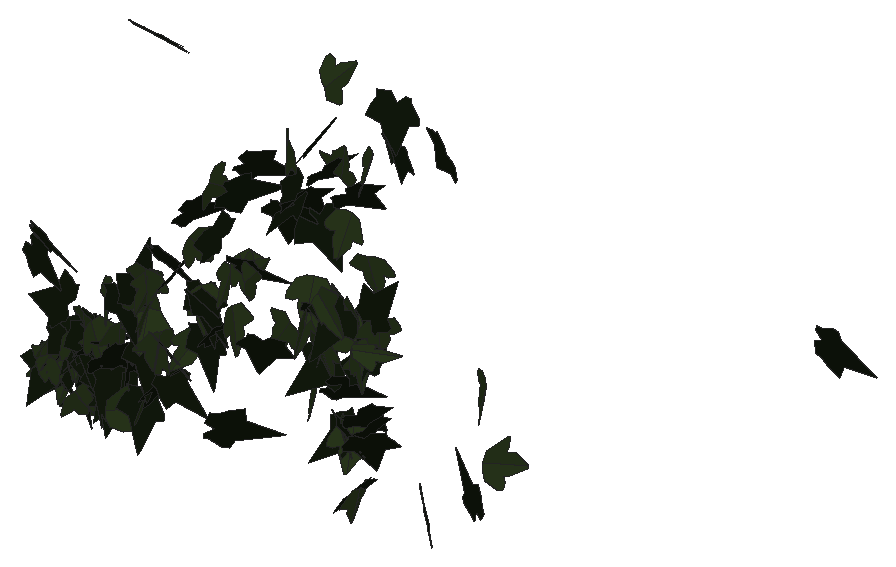
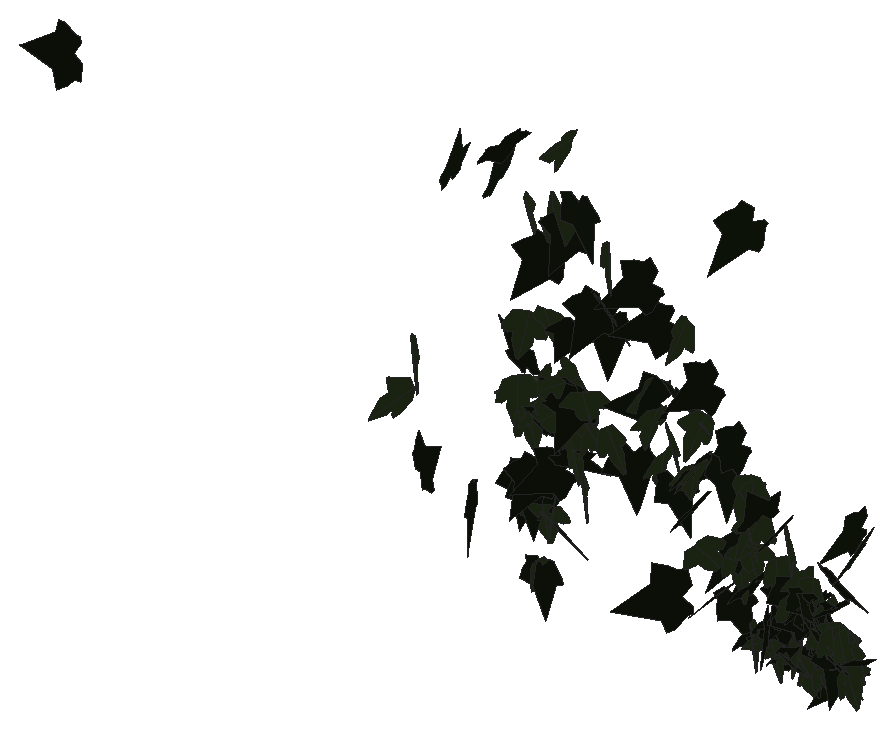
# SketchUp Ruby script. Lengths in inches.
U = 1.inch
M = Sketchup.active_model
def pt(a) = Geom::Point3d.new(a.map { |v| v * U })
def face(e, loops, mat)
  f = e.add_face(loops[0].map { |a| pt(a) })
  loops[1..].each { |l| e.add_face(l.map { |a| pt(a) }).erase! }
  f.material = f.back_material = mat if mat
  f
end
# faces: each face lists its corners as indices into pts; further lists are holes
def faces(e, pts, list, mat = nil) = list.each { |f| face(e, (f[0].is_a?(Array) ? f : [f]).map { |l| l.map { |i| pts[i] } }, mat) }
# xy, xz, yz: faces in a plane at the given z, y or x. An outline is a flat list of corners, or four numbers for a rectangle; further outlines are holes
def ring(l) = l.size == 4 ? [[l[0], l[1]], [l[2], l[1]], [l[2], l[3]], [l[0], l[3]]] : l.each_slice(2).to_a
def flat(e, list, mat, &to3) = list.each { |f| face(e, (f[0].is_a?(Array) ? f : [f]).map { |l| ring(l).map { |u, v| to3.(u, v) } }, mat) }
def xy(e, z, list, mat = nil) = flat(e, list, mat) { |x, y| [x, y, z] }
def xz(e, y, list, mat = nil) = flat(e, list, mat) { |x, z| [x, y, z] }
def yz(e, x, list, mat = nil) = flat(e, list, mat) { |y, z| [x, y, z] }
def lines(e, pts, list) = list.each { |a, b| e.add_line(pt(pts[a]), pt(pts[b])) }
# prism: a flat outline (further loops are holes) pulled along v
def prism(e, loops, v, mat = nil)
  f = face(e, loops, mat); d = Geom::Vector3d.new(v.map { |x| x * U })
  f.pushpull(f.normal.samedirection?(d) ? d.length : -d.length)
end
def box(e, o, s, mat = nil) = prism(e, [[o, [o[0] + s[0], o[1], o[2]], [o[0] + s[0], o[1] + s[1], o[2]], [o[0], o[1] + s[1], o[2]]]], [0, 0, s[2]], mat)
def at(x, y, z, deg = 0) = Geom::Transformation.translation(pt([x, y, z])) * Geom::Transformation.rotation(ORIGIN, Z_AXIS, deg.degrees)
def axes(o, x, y, z) = Geom::Transformation.new([*x, 0, *y, 0, *z, 0, *pt(o).to_a, 1])
def part(name) = M.definitions.add(name)
# library, detail: a bought-in or finely detailed component or shape, given as its bounding box
def library(name, o, s) = part(name).tap { |d| box(d.entities, o, s) }
def detail(e, o, s) = box(e.add_group.entities, o, s)
def put(e, d, t, mat = nil) = e.add_instance(d, t).tap { |i| i.material = mat if mat }
def group(e, t, mat = nil) = e.add_group.tap { |g| g.transformation = t; g.material = mat if mat }.entities
root = M.entities
M.materials.add("efeu1").color = [18, 25, 13]
M.materials.add("efeu2").color = [43, 57, 29]
c1 = part("ivyleaf_9")
p = [[1.54,2.16,1.25],[1.36,2.04,1.19],[-0.21,0.99,0.68],[-0.71,1.11,0.82],[-0.85,0.86,0.67],[-0.8,0.17,0.21],
  [-0.9,-0.01,0.1],[-0.67,-0.16,-0.02],[-0.08,-0.08,-0.05],[-0.03,-0.6,-0.4],[0.65,-0.88,-0.66],[0.83,-0.6,-0.49],
  [1.29,-0.42,-0.43],[1.8125,-0.07,-0.26],[1.21,0.44,0.15]]
faces(c1.entities,p,[[0,1,2,3,4,5,6,7,8,9,10,11,12,13,14]],"efeu1")
c2 = part("ivyleaf_10")
p = [[0,0.5,-0.03],[-0.0625,2.02,-0.43],[-0.19,2.01,-0.46],[-0.54,1.05,-0.29],[-0.52,0.625,-0.18],[-0.83,0.76,-0.28],
  [-1.16,0.64,-0.33],[-1.15,0.33,-0.24],[-0.77,-0.39,0.02],[-0.3,-0.51,0.16],[0.04,-0.48,0.23],[-0.02,2.01,-0.4375],
  [-0.06,2.01,-0.43],[0.04,-0.49,0.23],[0.67,-0.49,0.14],[1.38,0.36,-0.2],[1.375,0.51,-0.24],[0.81,0.65,-0.19],
  [0.62,0.59,-0.15],[0.6,1.09,-0.28],[0.5,1.23,-0.31]]
faces(c2.entities,p,[[0,1,2,3,4,5,6,7,8,9,10],[11,12,0,13,14,15,16,17,18,19,20]],"efeu2")
put(root,c1,axes([585.08,129.7,253.83],[1.04572,-0.05683,0.01946],[0.02203,0.04717,-1.04615],[0.05589,1.04484,0.04829]))
put(root,c2,axes([579.78,129.68,243.31],[-0.42415,-0.71462,-0.56248],[0.29905,0.47653,-0.83094],[0.85886,-0.51885,0.01155]))
put(root,c1,axes([587.74,130.46,249.34],[0.2356,-1.00803,0.0812],[0.02153,-0.07835,-1.03519],[1.01106,0.23656,0.00312]))
put(root,c2,axes([577.44,130.0625,244.39],[-0.84516,0.20624,0.52283],[-0.55979,-0.22451,-0.81634],[-0.05023,-0.96811,0.30069]))
put(root,c2,axes([595.76,130.15,254.29],[0.58897,0.00063,0.92492],[0.92487,0.01136,-0.58895],[-0.00992,1.09647,0.00557]))
put(root,c1,axes([592.11,129.78,250.8],[0.56686,0.68354,-0.59156],[-0.4325,-0.40807,-0.88596],[-0.7938,0.71046,0.06028]))
put(root,c1,axes([595.93,129.64,264.52],[-0.36405,1.05527,0.03181],[-0.00822,0.03081,-1.1163],[-1.05572,-0.36413,-0.00228]))
put(root,c2,axes([597.04,130.17,262.6],[-1.0381,0.08365,0.31829],[0.31731,-0.02495,1.04146],[0.08729,1.08551,-0.00059]))
put(root,c1,axes([578.63,130.28,246.41],[0.17103,-0.97793,-0.23774],[0.18827,0.26798,-0.96689],[0.98865,0.11815,0.22525]))
put(root,c2,axes([589.98,130.03,251.53],[-0.04841,1.04429,-0.13892],[0.00143,-0.13901,-1.0454],[-1.05349,-0.04818,0.00497]))
put(root,c2,axes([579.11,130.05,246.22],[0.0865,1.01039,-0.14055],[-0.02968,-0.13851,-1.01393],[-1.01968,0.08974,0.01759]))
put(root,c1,axes([584.63,129.36,267.26],[1.15865,0.34915,-0.23864],[-0.33283,0.32341,-1.14278],[-0.26092,1.13791,0.39802]))
put(root,c2,axes([580.74,129.8125,247.49],[0.01702,1.01449,0.18738],[-0.05066,0.188,-1.01325],[-1.0304,0.00751,0.05291]))
put(root,c2,axes([598.9,129.65,252.64],[0.66546,-0.78164,-0.07907],[0.78558,0.66311,0.05651],[0.00802,-0.09685,1.02499]))
put(root,c2,axes([583.99,130.6,251.39],[-0.01699,-0.87816,0.53969],[0.06668,-0.53957,-0.87586],[1.02858,0.02047,0.0657]))
put(root,c2,axes([588.93,129.52,259.43],[-0.03718,-0.63777,-0.85772],[0.11562,0.8508,-0.63764],[1.06257,-0.11489,0.03937]))
put(root,c1,axes([596.79,130.59,253.92],[-0.95992,-0.43922,-0.12493],[0.13077,0.01423,-1.05483],[0.43752,-0.96791,0.04118]))
put(root,c2,axes([584.14,130.0625,251.92],[-1.01434,-0.05409,0.16911],[-0.16615,-0.05661,-1.01469],[0.06259,-1.02678,0.04703]))
put(root,c1,axes([600.4,130.87,265.06],[0.17117,-0.7786,0.7468],[0.23075,-0.71222,-0.79544],[1.05389,0.2824,0.05287]))
put(root,c1,axes([576.52,129.99,250.92],[0.7137,-0.62816,-0.42994],[-0.25555,0.35743,-0.94643],[0.71702,0.75264,0.09063]))
put(root,c1,axes([581.13,130.66,244.72],[-0.24631,-0.97162,-0.0316],[0.00525,0.03127,-1.00235],[0.97212,-0.24635,-0.0026]))
put(root,c1,axes([596.55,129.41,262.91],[0.40146,0.95016,0.32318],[0.02996,0.33657,-1.02676],[-1.00317,0.39029,0.09867]))
put(root,c1,axes([582.04,130.47,249.91],[0.3517,-0.97481,-0.06017],[0.01617,0.06975,-1.03559],[0.97653,0.34992,0.03882]))
put(root,c1,axes([591.25,129.58,261.37],[0.80293,0.40631,0.56612],[0.51853,0.22863,-0.89952],[-0.46552,0.95547,-0.02549]))
put(root,c1,axes([599.04,129.8,247.32],[0.61441,0.79835,-0.297],[-0.17054,-0.2435,-1.00732],[-0.83456,0.63751,-0.01282]))
put(root,c2,axes([591.43,129.4,254.64],[0.10894,-0.01752,-1.05804],[0.07748,1.06091,-0.00959],[1.05534,-0.07608,0.10993]))
put(root,c1,axes([603.02,129.72,244.72],[0.473,-0.04615,-1.08266],[-1.05154,0.26586,-0.47074],[0.26181,1.15117,0.06531]))
put(root,c1,axes([587.52,130.37,251.75],[0.55737,-0.87545,-0.09952],[0.04791,0.14771,-1.03096],[0.87978,0.54658,0.1192]))
put(root,c1,axes([581.1,130.91,243.53],[-0.03524,-0.94211,0.37102],[0.07599,-0.37265,-0.93905],[1.00968,-0.00484,0.08362]))
put(root,c2,axes([583.86,130.29,249.78],[0.44977,-0.9049,-0.16697],[-0.09992,0.13672,-1.01012],[0.91474,0.45987,-0.02824]))
put(root,c1,axes([587.59,130.56,251.92],[0.19776,-1.00869,-0.13422],[-0.04239,0.12845,-1.02775],[1.01669,0.20156,-0.01675]))
put(root,c2,axes([598.74,130.37,263.73],[0.6375,-0.86934,-0.08392],[-0.05647,0.06265,-1.078],[0.87156,0.63994,-0.00847]))
put(root,c1,axes([590.33,130,254.66],[0.83608,-0.20903,0.61257],[0.63719,0.09002,-0.83896],[0.11371,1.03255,0.19715]))
put(root,c1,axes([590.18,129.49,259.35],[0.09954,0.53535,-0.92841],[0.13362,0.91894,0.54421],[1.06334,-0.16559,0.01853]))
put(root,c1,axes([588.97,130.07,255.82],[-0.64361,0.73023,0.38332],[-0.36076,0.18796,-0.96381],[-0.74164,-0.72514,0.13619]))
put(root,c1,axes([579.84,130.77,246.82],[-0.93479,-0.41363,-0.06479],[0.06117,0.02188,-1.0222],[0.41418,-0.93678,0.00474]))
put(root,c1,axes([579.65,130.76,246.53],[0.01366,-1.02388,-0.05878],[0.03218,0.05919,-1.02344],[1.02506,0.01178,0.03292]))
put(root,c1,axes([583.26,130.87,243.73],[-0.11947,-1.01271,0.05879],[-0.02267,-0.05652,-1.01961],[1.01416,-0.12056,-0.01587]))
put(root,c1,axes([576.6875,130.11,251.93],[0.96616,-0.36901,-0.14248],[-0.08239,0.18005,-1.02505],[0.38688,0.95987,0.1375]))
put(root,c1,axes([577.08,131.05,243.83],[-0.60378,-0.78567,0.20996],[0.02508,-0.27937,-0.97327],[0.81286,-0.57497,0.18599]))
put(root,c1,axes([578.55,130.1,248.2],[-0.61269,0.52484,0.67507],[-0.54767,0.39692,-0.80565],[-0.65668,-0.82071,0.04206]))
put(root,c1,axes([581.46,129.69,246.24],[0.39769,0.89977,0.25094],[0.12839,0.21749,-0.98333],[-0.92525,0.41692,-0.02859]))
put(root,c2,axes([581.14,130.5,249.875],[0.73225,-0.7306,0.07881],[0.15734,0.0472,-1.0243],[0.7178,0.73496,0.14412]))
put(root,c2,axes([587.62,130.35,251.8],[0.24925,1.00951,-0.07355],[-0.00894,-0.07355,-1.03979],[-1.01215,0.24925,-0.00893]))
put(root,c1,axes([589.03,130.15,250.5],[-0.22262,0.99718,-0.24179],[0.00178,-0.24704,-1.02046],[-1.02607,-0.21677,0.05069]))
put(root,c1,axes([596.99,131,246.5],[0.83591,-0.58108,-0.25404],[0.20113,-0.15571,1.01796],[-0.60145,-0.85968,-0.01266]))
put(root,c2,axes([581.96,130.4,247.83],[-0.11576,-0.99997,-0.13419],[0.02572,0.13211,-1.0066],[1.00861,-0.11813,0.01026]))
put(root,c2,axes([582.32,129.7,243.26],[-0.00009,0.02567,1.05537],[0.27659,1.0185,-0.02475],[-1.0188,0.27651,-0.00681]))
put(root,c1,axes([580.97,130.03,246.79],[0.19064,0.97908,-0.1769],[-0.13942,-0.15205,-0.9918],[-0.98511,0.21099,0.10614]))
put(root,c2,axes([589.08,130.53,253.38],[0.75306,-0.70421,-0.13856],[-0.08763,0.10911,-1.03084],[0.71234,0.75788,0.01966]))
put(root,c2,axes([598.07,130.45,252],[-0.09724,1.07,-0.13702],[-0.00038,-0.13761,-1.07433],[-1.07874,-0.09641,0.01273]))
put(root,c2,axes([593.25,130.47,251.82],[-0.80962,0.11397,0.63442],[-0.64457,-0.1419,-0.79708],[-0.00079,-1.01874,0.182]))
put(root,c2,axes([607.75,129.65,248.98],[-0.0138,0.37019,1.08543],[0.0478,1.08475,-0.36935],[-1.14583,0.04079,-0.02848]))
put(root,c2,axes([595.6,130.35,251.69],[-1.01493,0.36891,-0.06535],[0.07019,0.00184,-1.07959],[-0.36802,-1.01703,-0.02566]))
put(root,c1,axes([584.77,130.24,248.01],[0.98072,-0.12195,-0.2982],[-0.28528,0.11525,-0.98536],[0.1497,1.01855,0.07579]))
put(root,c1,axes([600.05,131.09,267.34],[-0.12461,-1.08112,-0.01233],[-0.01195,0.01379,-1.08819],[1.08112,-0.12446,-0.01345]))
put(root,c1,axes([586.94,129.75,256.83],[0.5554,0.58339,0.68873],[0.43171,0.53848,-0.80426],[-0.79266,0.70204,0.04456]))
put(root,c1,axes([598.84,130.54,254.29],[-0.43848,0.42566,0.83574],[0.59286,-0.58907,0.61108],[0.72674,0.73737,0.00573]))
put(root,c2,axes([595.02,130.41,248.59],[0.5666,-0.80732,-0.46619],[-0.1904,0.43383,-0.98269],[0.91261,0.59175,0.08442]))
put(root,c1,axes([593.67,130.8,260.04],[-1.01077,0.26582,-0.2538],[0.25317,-0.0348,-1.04471],[-0.26642,-1.04156,-0.02987]))
put(root,c2,axes([584.34,130.72,247.89],[-0.34429,-0.9639,0.0793],[0.0129,-0.08874,-1.02269],[0.96707,-0.34198,0.04187]))
put(root,c1,axes([583.28,131.15,246.66],[-0.0083,-1.00964,0.10048],[0.05512,-0.10078,-1.00814],[1.01313,-0.00279,0.05567]))
put(root,c1,axes([581.46,131.19,244.52],[-0.79135,-0.61537,-0.06535],[0.13678,-0.07047,-0.99273],[0.60352,-0.79091,0.1393]))
put(root,c2,axes([593.39,130.43,262.83],[-0.74157,0.68182,0.41174],[-0.46875,0.08124,-0.97878],[-0.64395,-0.84431,0.23832]))
put(root,c2,axes([580.41,130.77,246.36],[-0.60679,-0.79898,0.07098],[0.03091,-0.11223,-0.99902],[0.80153,-0.60053,0.09227]))
put(root,c2,axes([584.33,130.58,247.27],[0.95435,-0.2787,-0.22868],[-0.14035,0.30885,-0.96212],[0.33207,0.9315,0.25058]))
put(root,c2,axes([579.68,130.47,247.49],[-0.93793,0.25695,0.30351],[-0.2882,0.09654,-0.97236],[-0.27401,-0.98108,-0.01619]))
put(root,c2,axes([596.56,129.84,268.04],[0.31419,0.0398,-1.06146],[0.24978,1.07312,0.11417],[1.03242,-0.27174,0.2954]))
put(root,c1,axes([605.86,130.42,245.35],[0.20019,-0.34764,1.07436],[-0.47606,0.96343,0.40045],[-1.02395,-0.51589,0.02386]))
put(root,c1,axes([595.5625,131.31,250.19],[-0.91655,-0.39949,0.29446],[-0.24237,-0.17933,-0.99772],[0.43307,-0.94583,0.0648]))
put(root,c2,axes([598.28,130.93,251.625],[-0.25358,-0.98039,0.143],[-0.00711,-0.1458,-1.01223],[0.99074,-0.25197,0.02934]))
put(root,c1,axes([585.57,130.15,252.28],[-0.11669,0.97966,0.30334],[-0.0584,0.29845,-0.98634],[-1.02388,-0.12867,0.02168]))
put(root,c1,axes([583.18,130.38,250.29],[-0.40204,-0.45511,0.84782],[0.56212,0.63468,0.60726],[-0.78099,0.69109,0.00064]))
put(root,c1,axes([584.66,130.6875,245.35],[-0.31501,0.91287,-0.35343],[0.02637,-0.36323,-0.96169],[-0.97854,-0.30366,0.08786]))
put(root,c1,axes([593.16,130.5,258.88],[0.68214,0.61938,-0.57073],[-0.44049,-0.36362,-0.9211],[-0.71786,0.81168,0.02287]))
put(root,c2,axes([577.19,130.92,245.26],[0.1005,-1.01449,0.00003],[-0.00026,-0.00006,-1.01945],[1.01449,0.1005,-0.00027]))
put(root,c2,axes([594.01,131.19,252.24],[-0.17711,0.82011,-0.63695],[-0.12786,-0.65845,-0.81224],[-1.0305,-0.05925,0.21025]))
put(root,c2,axes([606.375,130.46,252.63],[0.58893,-0.76864,-0.74226],[-0.31589,0.68441,-0.95937],[1.02077,0.65526,0.13135]))
put(root,c1,axes([579.61,130.54,246.51],[-0.58031,0.83309,0.13215],[-0.08784,0.09985,-1.01517],[-0.83892,-0.58673,0.01487]))
put(root,c1,axes([579.89,130.42,246.79],[-0.1629,0.99353,0.02108],[-0.23397,-0.01758,-0.97931],[-0.96582,-0.16332,0.23368]))
put(root,c2,axes([576.6,131.08,243.53],[-0.04489,-0.98427,0.20514],[0.04594,-0.20714,-0.9838],[1.00437,-0.03451,0.05417]))
put(root,c1,axes([579.51,130.32,245.65],[-0.17386,0.96543,0.21213],[-0.04281,0.20783,-0.98094],[-0.98753,-0.17898,0.00518]))
put(root,c2,axes([577.77,130.95,245.36],[-0.32216,-0.96526,-0.00835],[0.02125,0.00171,-1.01741],[0.96506,-0.32226,0.01962]))
put(root,c2,axes([583.27,130.98,248.66],[0.87112,0.5145,-0.10846],[-0.08424,-0.07062,-1.01156],[-0.51902,0.875,-0.01787]))
put(root,c2,axes([583.2,130.88,243.68],[0.45678,-0.8954,-0.18049],[0.00367,0.2036,-1.00075],[0.9134,0.44696,0.09429]))
put(root,c2,axes([578.14,130.91,245.48],[-0.75809,-0.66342,0.07731],[-0.0695,-0.03795,-1.00724],[0.66428,-0.76107,-0.01716]))
put(root,c1,axes([578.68,131.21,243.34],[-0.16762,-0.00421,-0.99195],[0.99145,-0.03292,-0.16739],[-0.03176,-1.00548,0.00963]))
put(root,c2,axes([577.97,131.33,243.65],[-0.27782,-0.86274,0.42387],[0.09954,-0.46466,-0.88053],[0.95607,-0.20232,0.21485]))
put(root,c1,axes([585.05,130.68,245.74],[0.63865,-0.65268,-0.47691],[-0.0315,0.58723,-0.84585],[0.80774,0.53895,0.34408]))
put(root,c1,axes([577.92,131.16,244],[-0.98863,0.10593,-0.05742],[0.05988,0.02006,-0.99395],[-0.10456,-0.9901,-0.02628]))
put(root,c1,axes([580.58,131.51,243.43],[-0.78322,-0.30522,0.54424],[-0.47995,-0.26347,-0.83846],[0.39875,-0.91664,0.05978]))
put(root,c1,axes([598.48,130.54,251.07],[-0.99496,0.20598,-0.10675],[-0.1042,0.02324,1.01606],[0.20728,1.0004,-0.00163]))
put(root,c2,axes([596.7,131.27,252.08],[0.44996,0.46369,0.83106],[-0.57505,-0.59999,0.64611],[0.75828,-0.73016,-0.00316]))
put(root,c2,axes([589.96,130.76,254.37],[0.11445,1.02913,0.14036],[-0.00471,0.14172,-1.03528],[-1.03865,0.11276,0.02016]))
put(root,c2,axes([583.14,130.71,250.21],[-0.5539,-0.69585,-0.51256],[0.3226,0.39832,-0.88938],[0.80178,-0.64098,0.00375]))
put(root,c2,axes([596.91,130.64,246.62],[-0.64515,0.5733,0.50596],[-0.40764,0.3022,-0.8622],[-0.64692,-0.76216,0.03872]))
put(root,c2,axes([587.05,130.4,254.77],[0.26681,0.74564,0.68177],[-0.19181,0.7297,-0.72299],[-0.99196,0.05946,0.32317]))
put(root,c1,axes([602.79,131.83,264.97],[-0.18605,-0.44322,0.99252],[0.23071,-1.00012,-0.40336],[1.06222,0.13959,0.26145]))
put(root,c1,axes([597.43,130.35,261.36],[0.71277,0.76299,0.25695],[0.1645,0.19791,-1.04402],[-0.78811,0.73136,0.01446]))
put(root,c1,axes([598.29,130.62,247.27],[0.00491,1.02644,-0.04252],[-0.00257,-0.0425,-1.02645],[-1.02731,0.00501,0.00236]))
put(root,c2,axes([596.97,131.14,246.33],[0.97588,0.38067,-0.02341],[-0.02073,-0.01128,-1.04749],[-0.38083,0.97609,-0.00297]))
put(root,c2,axes([598.4375,131.02,257.24],[-1.0352,-0.15617,-0.05421],[0.05423,0.00395,-1.04691],[0.15617,-1.03661,0.00418]))
put(root,c2,axes([597.2,130.89,253.53],[-0.49766,0.25021,-0.8928],[-0.76579,0.46035,0.55588],[0.52274,0.91259,-0.03563]))
put(root,c1,axes([579.27,131.11,246.29],[0.85122,-0.33682,0.41046],[0.40822,-0.08081,-0.91287],[0.33954,0.94156,0.06849]))
put(root,c1,axes([577.2,131.11,243.21],[0.86809,-0.46822,-0.09834],[-0.07938,0.05995,-0.98619],[0.4718,0.87158,0.015]))
put(root,c1,axes([597.92,130.61,248.09],[0.5997,0.79696,0.14631],[0.07747,0.1248,-0.9973],[-0.80656,0.60454,0.01299]))
put(root,c1,axes([580.42,131.4,243.39],[-0.88914,0.45497,0.07745],[-0.16289,-0.15206,-0.97668],[-0.43182,-0.87946,0.20894]))
put(root,c2,axes([594.11,131.35,254.2],[0.87301,0.56369,-0.10968],[-0.08385,-0.07232,-1.03907],[-0.56811,0.87689,-0.01519]))
put(root,c1,axes([595.11,130.77,253.55],[0.82896,0.62198,-0.21562],[-0.24708,-0.0274,-1.02894],[-0.61016,0.85611,0.12372]))
put(root,c1,axes([588.41,130.62,243.93],[0.85113,0.31971,0.86466],[0.81236,0.29622,-0.90918],[-0.4358,1.17657,-0.00606]))
put(root,c2,axes([586.14,131.61,248.03],[0.57558,0.55557,-0.6352],[-0.51699,-0.37555,-0.79693],[-0.66697,0.77054,0.06957]))
put(root,c2,axes([597.1875,131.44,242.81],[0.08365,-0.98048,-0.00849],[-0.00901,0.00775,-0.98401],[0.98047,0.08372,-0.00831]))
put(root,c1,axes([577.48,130.75,244.25],[0.14534,0.99306,0.14389],[0.04209,0.13923,-1.00341],[-1.00254,0.14981,-0.02127]))
put(root,c2,axes([578.55,131.47,242.625],[-0.53483,-0.02065,0.83927],[0.83952,-0.01294,0.53467],[-0.00018,0.99511,0.02437]))
put(root,c1,axes([596.41,131.55,246.22],[-0.98865,0.2778,-0.01695],[0.00019,-0.06187,-1.02521],[-0.27832,-0.98685,0.05951]))
put(root,c2,axes([598.71,131.35,253.39],[-0.61173,-0.82624,-0.05911],[0.04416,0.04085,-1.02799],[0.82717,-0.61322,0.01116]))
put(root,c1,axes([593.72,130.71,259.54],[0.5586,0.89293,0.21313],[0.12262,0.17468,-1.0532],[-0.90979,0.57179,-0.01109]))
put(root,c1,axes([628.6875,131.39,262.92],[0.41719,0.16085,-1.15793],[1.05248,0.48349,0.44636],[0.50887,-1.13185,0.02611]))
put(root,c1,axes([596.02,130.9,249.02],[0.8254,0.3655,0.52651],[0.45169,0.27736,-0.90063],[-0.45474,0.93892,0.06109]))
put(root,c1,axes([594.61,131.53,258.5],[-0.24848,-0.71957,-0.74613],[0.2896,0.68852,-0.76046],[0.9953,-0.37998,0.035]))
put(root,c2,axes([581.24,131.54,243.87],[0.91926,-0.36909,-0.14474],[-0.08323,0.17768,-0.9817],[0.38762,0.91347,0.13247]))
put(root,c2,axes([594.71,131.625,251.22],[0.26879,-0.99845,-0.0849],[-0.03333,0.07894,-1.03393],[1.0015,0.2706,-0.01162]))
put(root,c1,axes([597.15,131.14,242.87],[-0.07121,0.98284,0.02322],[-0.01401,0.02226,-0.98534],[-0.98301,-0.07151,0.01237]))
put(root,c2,axes([579.78,131.375,244.62],[-0.75872,0.61214,0.2255],[-0.20078,0.10997,-0.97407],[-0.62069,-0.78384,0.03944]))
put(root,c2,axes([596.2,131.74,258.61],[1.05949,-0.11215,-0.11915],[-0.11825,0.01476,-1.06541],[0.11309,1.06607,0.00222]))
put(root,c1,axes([581.93,131.2,245.07],[0.08361,0.02228,-1.00472],[-0.89355,0.46305,-0.06409],[0.45993,0.89557,0.05813]))
